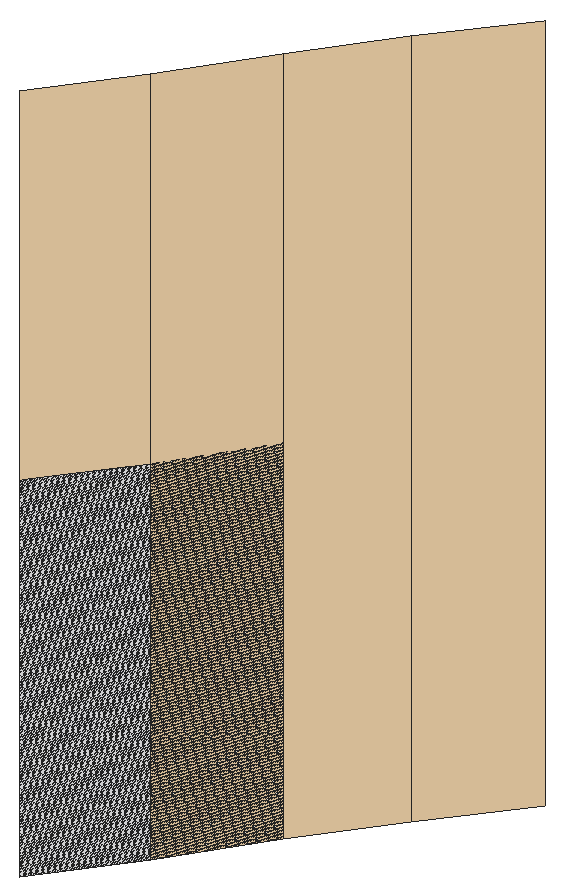
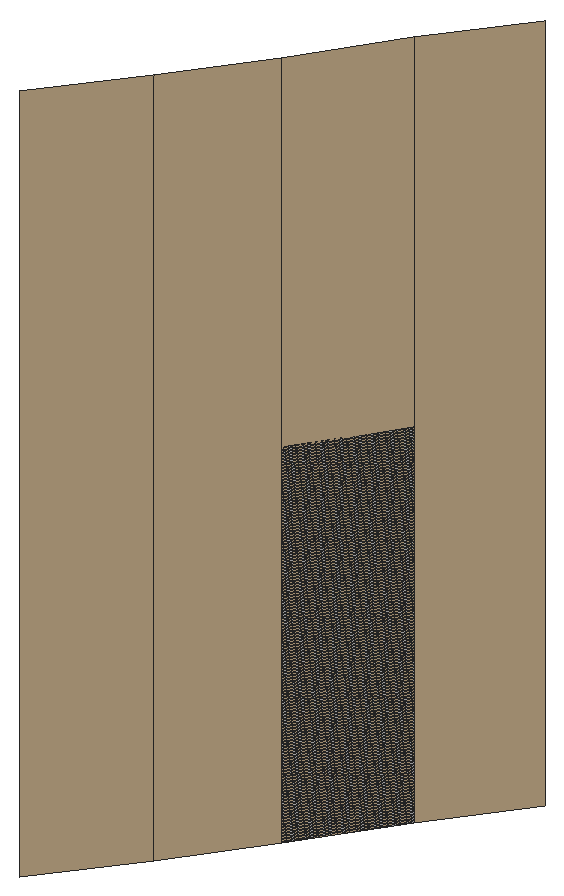
# SketchUp Ruby script. Lengths in inches.
U = 1.inch
M = Sketchup.active_model
def pt(a) = Geom::Point3d.new(a.map { |v| v * U })
def face(e, loops, mat)
  f = e.add_face(loops[0].map { |a| pt(a) })
  loops[1..].each { |l| e.add_face(l.map { |a| pt(a) }).erase! }
  f.material = f.back_material = mat if mat
  f
end
# faces: each face lists its corners as indices into pts; further lists are holes
def faces(e, pts, list, mat = nil) = list.each { |f| face(e, (f[0].is_a?(Array) ? f : [f]).map { |l| l.map { |i| pts[i] } }, mat) }
# xy, xz, yz: faces in a plane at the given z, y or x. An outline is a flat list of corners, or four numbers for a rectangle; further outlines are holes
def ring(l) = l.size == 4 ? [[l[0], l[1]], [l[2], l[1]], [l[2], l[3]], [l[0], l[3]]] : l.each_slice(2).to_a
def flat(e, list, mat, &to3) = list.each { |f| face(e, (f[0].is_a?(Array) ? f : [f]).map { |l| ring(l).map { |u, v| to3.(u, v) } }, mat) }
def xy(e, z, list, mat = nil) = flat(e, list, mat) { |x, y| [x, y, z] }
def xz(e, y, list, mat = nil) = flat(e, list, mat) { |x, z| [x, y, z] }
def yz(e, x, list, mat = nil) = flat(e, list, mat) { |y, z| [x, y, z] }
def lines(e, pts, list) = list.each { |a, b| e.add_line(pt(pts[a]), pt(pts[b])) }
# prism: a flat outline (further loops are holes) pulled along v
def prism(e, loops, v, mat = nil)
  f = face(e, loops, mat); d = Geom::Vector3d.new(v.map { |x| x * U })
  f.pushpull(f.normal.samedirection?(d) ? d.length : -d.length)
end
def box(e, o, s, mat = nil) = prism(e, [[o, [o[0] + s[0], o[1], o[2]], [o[0] + s[0], o[1] + s[1], o[2]], [o[0], o[1] + s[1], o[2]]]], [0, 0, s[2]], mat)
def at(x, y, z, deg = 0) = Geom::Transformation.translation(pt([x, y, z])) * Geom::Transformation.rotation(ORIGIN, Z_AXIS, deg.degrees)
def axes(o, x, y, z) = Geom::Transformation.new([*x, 0, *y, 0, *z, 0, *pt(o).to_a, 1])
def part(name) = M.definitions.add(name)
# library, detail: a bought-in or finely detailed component or shape, given as its bounding box
def library(name, o, s) = part(name).tap { |d| box(d.entities, o, s) }
def detail(e, o, s) = box(e.add_group.entities, o, s)
def put(e, d, t, mat = nil) = e.add_instance(d, t).tap { |i| i.material = mat if mat }
def group(e, t, mat = nil) = e.add_group.tap { |g| g.transformation = t; g.material = mat if mat }.entities
root = M.entities
M.materials.add("False Ceiling Light").color = [254, 223, 179]
M.materials.add("[Quartz Light Grey]").color = [251, 251, 252]
p = [[45.875,211.65,115.32],[45.98,211.79,115.32],[45.98,211.79,116.49],[45.875,211.65,116.49],[45.98,211.79,115.32],[45.875,211.65,115.32],
  [45.875,211.65,115.91],[45.98,211.79,115.91],[46.08,211.94,115.32],[46.08,211.94,116.49],[46.08,211.94,115.32],[46.08,211.94,115.91],
  [46.18,212.08,115.32],[46.18,212.08,116.49],[46.18,212.08,115.32],[46.18,212.08,115.91],[46.29,212.22,115.32],[46.29,212.22,116.49]]
faces(root,p,[[0,1,2,3],[1,8,9,2],[8,12,13,9],[12,16,17,13]],"False Ceiling Light")
faces(root,p,[[4,5,6,7],[10,4,7,11],[14,10,11,15]],"[Quartz Light Grey]")
